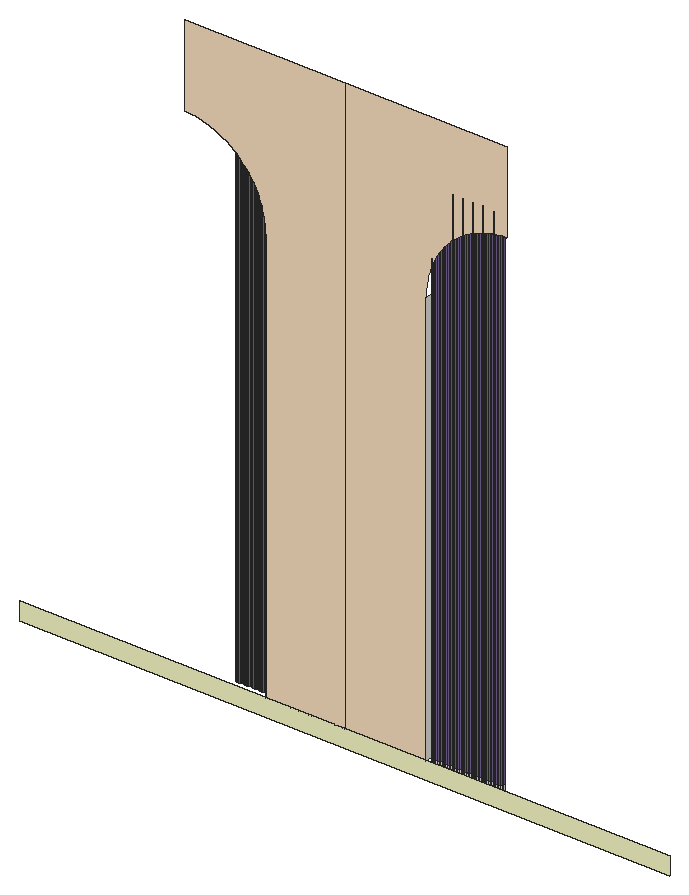
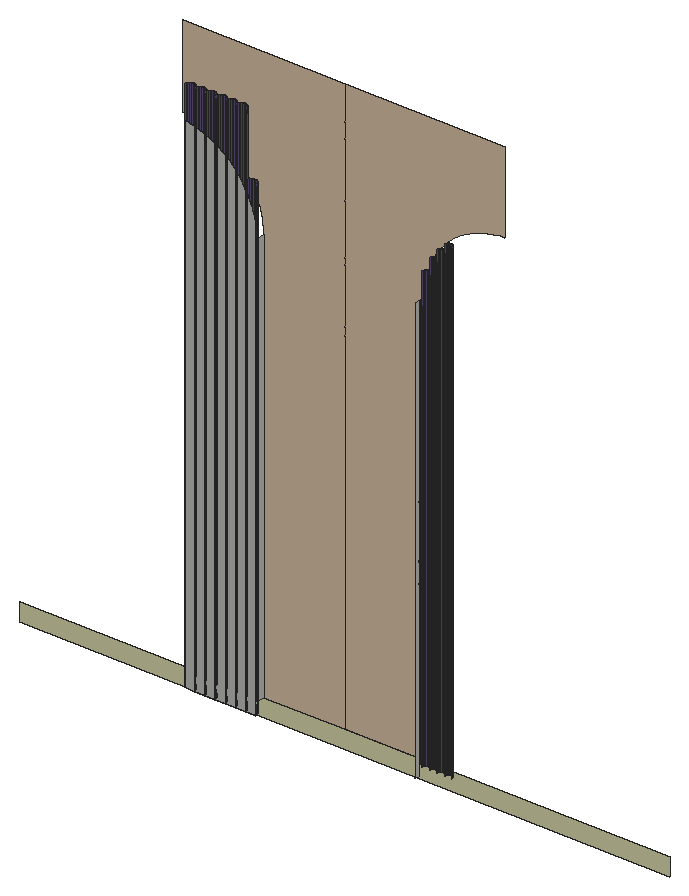
# SketchUp Ruby script. Lengths in inches.
U = 1.inch
M = Sketchup.active_model
def pt(a) = Geom::Point3d.new(a.map { |v| v * U })
def face(e, loops, mat)
  f = e.add_face(loops[0].map { |a| pt(a) })
  loops[1..].each { |l| e.add_face(l.map { |a| pt(a) }).erase! }
  f.material = f.back_material = mat if mat
  f
end
# faces: each face lists its corners as indices into pts; further lists are holes
def faces(e, pts, list, mat = nil) = list.each { |f| face(e, (f[0].is_a?(Array) ? f : [f]).map { |l| l.map { |i| pts[i] } }, mat) }
# xy, xz, yz: faces in a plane at the given z, y or x. An outline is a flat list of corners, or four numbers for a rectangle; further outlines are holes
def ring(l) = l.size == 4 ? [[l[0], l[1]], [l[2], l[1]], [l[2], l[3]], [l[0], l[3]]] : l.each_slice(2).to_a
def flat(e, list, mat, &to3) = list.each { |f| face(e, (f[0].is_a?(Array) ? f : [f]).map { |l| ring(l).map { |u, v| to3.(u, v) } }, mat) }
def xy(e, z, list, mat = nil) = flat(e, list, mat) { |x, y| [x, y, z] }
def xz(e, y, list, mat = nil) = flat(e, list, mat) { |x, z| [x, y, z] }
def yz(e, x, list, mat = nil) = flat(e, list, mat) { |y, z| [x, y, z] }
def lines(e, pts, list) = list.each { |a, b| e.add_line(pt(pts[a]), pt(pts[b])) }
# prism: a flat outline (further loops are holes) pulled along v
def prism(e, loops, v, mat = nil)
  f = face(e, loops, mat); d = Geom::Vector3d.new(v.map { |x| x * U })
  f.pushpull(f.normal.samedirection?(d) ? d.length : -d.length)
end
def box(e, o, s, mat = nil) = prism(e, [[o, [o[0] + s[0], o[1], o[2]], [o[0] + s[0], o[1] + s[1], o[2]], [o[0], o[1] + s[1], o[2]]]], [0, 0, s[2]], mat)
def at(x, y, z, deg = 0) = Geom::Transformation.translation(pt([x, y, z])) * Geom::Transformation.rotation(ORIGIN, Z_AXIS, deg.degrees)
def axes(o, x, y, z) = Geom::Transformation.new([*x, 0, *y, 0, *z, 0, *pt(o).to_a, 1])
def part(name) = M.definitions.add(name)
# library, detail: a bought-in or finely detailed component or shape, given as its bounding box
def library(name, o, s) = part(name).tap { |d| box(d.entities, o, s) }
def detail(e, o, s) = box(e.add_group.entities, o, s)
def put(e, d, t, mat = nil) = e.add_instance(d, t).tap { |i| i.material = mat if mat }
def group(e, t, mat = nil) = e.add_group.tap { |g| g.transformation = t; g.material = mat if mat }.entities
root = M.entities
M.materials.add("[0012_Bisque]").color = [255, 228, 196]
M.materials.add("[Color E01]").color = [255, 255, 204]
M.materials.add("[Color I01]").color = [116, 98, 147]
xy(root,5.5,[[176.942,140.478,176.756,140.503,176.583,140.575,176.434,140.689,176.32,140.838,176.248,141.011,176.224,141.197,177.661,141.197,177.637,141.011,177.565,140.838,177.451,140.689,177.302,140.575,177.128,140.503],[178.38,140.478,178.194,140.503,178.02,140.575,177.872,140.689,177.757,140.838,177.686,141.011,177.661,141.197,179.099,141.197,179.074,141.011,179.002,140.838,178.888,140.689,178.739,140.575,178.566,140.503],[179.817,140.478,179.631,140.503,179.458,140.575,179.309,140.689,179.195,140.838,179.123,141.011,179.099,141.197,180.536,141.197,180.512,141.011,180.44,140.838,180.326,140.689,180.177,140.575,180.003,140.503],[181.255,140.478,181.069,140.503,180.895,140.575,180.747,140.689,180.632,140.838,180.561,141.011,180.536,141.197,181.974,141.197,181.949,141.011,181.877,140.838,181.763,140.689,181.614,140.575,181.441,140.503],[182.692,140.478,182.506,140.503,182.333,140.575,182.184,140.689,182.07,140.838,181.998,141.011,181.974,141.197,183.411,141.197,183.387,141.011,183.315,140.838,183.201,140.689,183.052,140.575,182.878,140.503],
  [184.13,140.478,183.944,140.503,183.77,140.575,183.622,140.689,183.507,140.838,183.436,141.011,183.411,141.197,184.849,141.197,184.824,141.011,184.752,140.838,184.638,140.689,184.489,140.575,184.316,140.503],[185.567,140.478,185.381,140.503,185.208,140.575,185.059,140.689,184.945,140.838,184.873,141.011,184.849,141.197,186.286,141.197,186.262,141.011,186.19,140.838,186.076,140.689,185.927,140.575,185.753,140.503],[153.72,140.735,153.724,140.737,153.834,140.822,153.918,140.932,153.971,141.06,153.989,141.197,153.72,141.197]])
xz(root,139.885,[[153.72,7.1875,164.816,7.1875,164.816,88.4375,142.302,88.4375,142.302,76.971,142.307,76.971,142.612,76.963,142.917,76.947,143.221,76.923,143.525,76.891,143.828,76.851,144.129,76.803,144.429,76.747,144.728,76.683,145.024,76.611,145.319,76.531,145.612,76.444,145.902,76.349,146.189,76.246,146.474,76.136,146.756,76.018,147.034,75.893,147.309,75.761,147.581,75.621,147.848,75.474,148.112,75.321,148.372,75.16,148.627,74.993,148.878,74.818,149.124,74.638,149.365,74.451,149.601,74.257,149.832,74.058,150.058,73.852,150.278,73.64,150.492,73.423,150.701,73.2,150.904,72.972,151.1,72.738,151.291,72.5,151.475,72.256,151.652,72.008,151.823,71.755,151.987,71.497,152.145,71.236,152.295,70.97,152.438,70.7,152.574,70.427,152.703,70.15,152.825,69.87,152.939,69.587,153.045,69.301,153.144,69.012,153.235,68.721,153.319,68.427,153.395,68.132,153.463,67.834,153.523,67.535,153.575,67.234,153.619,66.932,153.655,66.629,153.683,66.325,153.704,66.02,153.716,65.715,153.72,65.41],[164.816,7.1875,176.224,7.1875,176.224,65.41,176.228,65.71,176.239,66.01,176.259,66.309,176.286,66.608,176.321,66.906,176.364,67.203,176.414,67.499,176.472,67.793,176.538,68.086,176.611,68.377,176.692,68.666,176.78,68.953,176.876,69.237,176.979,69.519,177.089,69.798,177.206,70.075,177.331,70.348,177.463,70.617,177.601,70.883,177.747,71.146,177.899,71.405,178.058,71.659,178.224,71.909,178.395,72.155,178.574,72.397,178.758,72.634,178.949,72.865,179.145,73.092,179.347,73.314,179.555,73.53,179.769,73.741,179.988,73.946,180.212,74.146,180.441,74.34,180.676,74.527,180.915,74.709,181.158,74.884,181.406,75.053,181.659,75.215,181.915,75.371,182.176,75.52,182.44,75.662,182.708,75.797,182.979,75.926,183.254,76.047,183.531,76.161,183.812,76.268,184.095,76.367,184.381,76.459,184.669,76.544,184.959,76.621,185.25,76.691,185.544,76.753,185.839,76.807,186.136,76.854,186.433,76.893,186.732,76.924,187.031,76.947,187.331,76.963,187.631,76.952,187.631,88.4375,164.816,88.4375]],"[0012_Bisque]")
xz(root,139.885,[[119.1875,4.6875,210.445,7.1875]],"[Color E01]")
xz(root,141.197,[[176.224,5.5,177.661,5.5,177.661,70.991,177.601,70.883,177.463,70.617,177.331,70.348,177.206,70.075,177.089,69.798,176.979,69.519,176.876,69.237,176.78,68.953,176.692,68.666,176.611,68.377,176.538,68.086,176.472,67.793,176.414,67.499,176.364,67.203,176.321,66.906,176.286,66.608,176.259,66.309,176.239,66.01,176.228,65.71,176.224,65.41],[177.661,5.5,177.661,70.991,177.747,71.146,177.899,71.405,178.058,71.659,178.224,71.909,178.395,72.155,178.574,72.397,178.758,72.634,178.949,72.865,179.099,73.039,179.099,5.5],[179.099,5.5,180.536,5.5,180.536,74.416,180.441,74.34,180.212,74.146,179.988,73.946,179.769,73.741,179.555,73.53,179.347,73.314,179.145,73.092,179.099,73.039],[180.536,5.5,181.974,5.5,181.974,75.404,181.915,75.371,181.659,75.215,181.406,75.053,181.158,74.884,180.915,74.709,180.676,74.527,180.536,74.416],[181.974,5.5,183.411,5.5,183.411,76.111,183.254,76.047,182.979,75.926,182.708,75.797,182.44,75.662,182.176,75.52,181.974,75.404],
  [183.411,5.5,184.849,5.5,184.849,76.592,184.669,76.544,184.381,76.459,184.095,76.367,183.812,76.268,183.531,76.161,183.411,76.111],[184.849,5.5,186.286,5.5,186.286,76.873,186.136,76.854,185.839,76.807,185.544,76.753,185.25,76.691,184.959,76.621,184.849,76.592]])
yz(root,153.72,[[140.735,5.5,141.197,65.41],[139.885,7.1875,140.735,65.41]])
yz(root,176.224,[[139.885,7.1875,141.197,65.41]])
p = [[176.583,140.575,5.5],[176.756,140.503,5.5],[176.756,140.503,7.1875],[176.583,140.575,7.1875],[176.942,140.478,5.5],[176.942,140.478,7.1875],
  [177.128,140.503,5.5],[177.128,140.503,7.1875],[177.302,140.575,5.5],[177.302,140.575,7.1875],[178.02,140.575,5.5],[178.194,140.503,5.5],
  [178.194,140.503,7.1875],[178.02,140.575,7.1875],[178.38,140.478,5.5],[178.38,140.478,7.1875],[178.566,140.503,5.5],[178.566,140.503,7.1875],
  [178.739,140.575,5.5],[178.739,140.575,7.1875],[179.458,140.575,5.5],[179.631,140.503,5.5],[179.631,140.503,7.1875],[179.458,140.575,7.1875],
  [179.817,140.478,5.5],[179.817,140.478,7.1875],[180.003,140.503,5.5],[180.003,140.503,7.1875],[180.177,140.575,5.5],[180.177,140.575,7.1875],
  [180.895,140.575,5.5],[181.069,140.503,5.5],[181.069,140.503,7.1875],[180.895,140.575,7.1875],[181.255,140.478,5.5],[181.255,140.478,7.1875],
  [181.441,140.503,5.5],[181.441,140.503,7.1875],[181.614,140.575,5.5],[181.614,140.575,7.1875],[182.333,140.575,5.5],[182.506,140.503,5.5],
  [182.506,140.503,7.1875],[182.333,140.575,7.1875],[182.692,140.478,5.5],[182.692,140.478,7.1875],[182.878,140.503,5.5],[182.878,140.503,7.1875],
  [183.052,140.575,5.5],[183.052,140.575,7.1875],[183.77,140.575,5.5],[183.944,140.503,5.5],[183.944,140.503,7.1875],[183.77,140.575,7.1875],
  [184.13,140.478,5.5],[184.13,140.478,7.1875],[184.316,140.503,5.5],[184.316,140.503,7.1875],[184.489,140.575,5.5],[184.489,140.575,7.1875],
  [185.208,140.575,5.5],[185.381,140.503,5.5],[185.381,140.503,7.1875],[185.208,140.575,7.1875],[185.567,140.478,5.5],[185.567,140.478,7.1875],
  [185.753,140.503,5.5],[185.753,140.503,7.1875],[185.927,140.575,5.5],[185.927,140.575,7.1875],[176.434,140.689,5.5],[176.434,140.689,7.1875],
  [177.451,140.689,5.5],[177.451,140.689,7.1875],[177.872,140.689,5.5],[177.872,140.689,7.1875],[178.888,140.689,5.5],[178.888,140.689,7.1875],
  [179.309,140.689,5.5],[179.309,140.689,7.1875],[180.326,140.689,5.5],[180.326,140.689,7.1875],[180.747,140.689,5.5],[180.747,140.689,7.1875],
  [181.763,140.689,5.5],[181.763,140.689,7.1875],[182.184,140.689,5.5],[182.184,140.689,7.1875],[183.201,140.689,5.5],[183.201,140.689,7.1875],
  [183.622,140.689,5.5],[183.622,140.689,7.1875],[184.638,140.689,5.5],[184.638,140.689,7.1875],[185.059,140.689,5.5],[185.059,140.689,7.1875],
  [186.076,140.689,5.5],[186.076,140.689,7.1875],[176.32,140.838,5.5],[176.32,140.838,7.1875],[177.565,140.838,5.5],[177.565,140.838,7.1875],
  [177.757,140.838,5.5],[177.757,140.838,7.1875],[179.002,140.838,5.5],[179.002,140.838,7.1875],[179.195,140.838,5.5],[179.195,140.838,7.1875],
  [180.44,140.838,5.5],[180.44,140.838,7.1875],[180.632,140.838,5.5],[180.632,140.838,7.1875],[181.877,140.838,5.5],[181.877,140.838,7.1875],
  [182.07,140.838,5.5],[182.07,140.838,7.1875],[183.315,140.838,5.5],[183.315,140.838,7.1875],[183.507,140.838,5.5],[183.507,140.838,7.1875],
  [184.752,140.838,5.5],[184.752,140.838,7.1875],[184.945,140.838,5.5],[184.945,140.838,7.1875],[186.19,140.838,5.5],[186.19,140.838,7.1875],
  [176.248,141.011,7.1875],[176.248,141.011,5.5],[177.637,141.011,5.5],[177.637,141.011,7.1875],[177.686,141.011,5.5],[177.686,141.011,7.1875],
  [179.074,141.011,5.5],[179.074,141.011,7.1875],[179.123,141.011,5.5],[179.123,141.011,7.1875],[180.512,141.011,5.5],[180.512,141.011,7.1875],
  [180.561,141.011,5.5],[180.561,141.011,7.1875],[181.949,141.011,5.5],[181.949,141.011,7.1875],[181.998,141.011,5.5],[181.998,141.011,7.1875],
  [183.387,141.011,5.5],[183.387,141.011,7.1875],[183.436,141.011,5.5],[183.436,141.011,7.1875],[184.824,141.011,5.5],[184.824,141.011,7.1875],
  [184.873,141.011,5.5],[184.873,141.011,7.1875],[186.262,141.011,5.5],[186.262,141.011,7.1875],[176.224,141.197,5.5],[176.224,141.197,7.1875],
  [177.661,141.197,5.5],[177.661,141.197,7.1875],[179.099,141.197,5.5],[179.099,141.197,7.1875],[180.536,141.197,5.5],[180.536,141.197,7.1875],
  [181.974,141.197,5.5],[181.974,141.197,7.1875],[183.411,141.197,5.5],[183.411,141.197,7.1875],[184.849,141.197,5.5],[184.849,141.197,7.1875],
  [186.286,141.197,5.5],[186.286,141.197,7.1875],[176.583,140.575,72.397],[176.756,140.503,72.397],[176.942,140.478,72.397],[177.128,140.503,72.397],
  [177.302,140.575,72.397],[178.02,140.575,81.5],[178.194,140.503,81.5],[178.38,140.478,81.5],[178.566,140.503,81.5],[178.739,140.575,81.5],
  [179.458,140.575,81.5],[179.631,140.503,81.5],[179.817,140.478,81.5],[180.003,140.503,81.5],[180.177,140.575,81.5],[180.895,140.575,81.5],
  [181.069,140.503,81.5],[181.255,140.478,81.5],[181.441,140.503,81.5],[181.614,140.575,81.5],[182.333,140.575,81.5],[182.506,140.503,81.5],
  [182.692,140.478,81.5],[182.878,140.503,81.5],[183.052,140.575,81.5],[183.77,140.575,81.5],[183.944,140.503,81.5],[184.13,140.478,81.5],
  [184.316,140.503,81.5],[184.489,140.575,81.5],[185.208,140.575,81.5],[185.381,140.503,81.5],[185.567,140.478,81.5],[185.753,140.503,81.5],
  [185.927,140.575,81.5],[176.434,140.689,72.397],[177.451,140.689,72.397],[177.872,140.689,81.5],[178.888,140.689,81.5],[179.309,140.689,81.5],
  [180.326,140.689,81.5],[180.747,140.689,81.5],[181.763,140.689,81.5],[182.184,140.689,81.5],[183.201,140.689,81.5],[183.622,140.689,81.5],
  [184.638,140.689,81.5],[185.059,140.689,81.5],[186.076,140.689,81.5],[148.833,140.822,74.138],[148.833,140.822,7.1875],[148.943,140.737,7.1875],
  [148.943,140.737,74.138],[149.071,140.684,7.1875],[149.071,140.684,74.138],[149.208,140.666,7.1875],[149.208,140.666,74.138],[149.346,140.684,7.1875],
  [149.346,140.684,74.138],[149.474,140.737,7.1875],[149.474,140.737,74.138],[149.584,140.822,7.1875],[149.584,140.822,74.138],[149.895,140.822,73.087],
  [149.895,140.822,7.1875],[150.005,140.737,7.1875],[150.005,140.737,73.087],[150.133,140.684,7.1875],[150.133,140.684,73.087],[150.271,140.666,7.1875],
  [150.271,140.666,73.087],[150.408,140.684,7.1875],[150.408,140.684,73.087],[150.536,140.737,7.1875],[150.536,140.737,73.087],[150.646,140.822,7.1875],
  [150.646,140.822,73.087],[150.958,140.822,71.69],[150.958,140.822,7.1875],[151.068,140.737,7.1875],[151.068,140.737,71.69],[151.196,140.684,7.1875],
  [151.196,140.684,71.69],[151.333,140.666,7.1875],[151.333,140.666,71.69],[151.471,140.684,7.1875],[151.471,140.684,71.69],[151.599,140.737,7.1875],
  [151.599,140.737,71.69],[151.709,140.822,7.1875],[151.709,140.822,71.69],[152.02,140.822,69.616],[152.02,140.822,7.1875],[152.13,140.737,7.1875],
  [152.13,140.737,69.616],[152.258,140.684,7.1875],[152.258,140.684,69.616],[152.396,140.666,7.1875],[152.396,140.666,69.616],[152.533,140.684,7.1875],
  [152.533,140.684,69.616],[152.661,140.737,7.1875],[152.661,140.737,69.616],[152.771,140.822,7.1875],[152.771,140.822,69.616],[153.083,140.822,65.41],
  [153.083,140.822,7.1875],[153.193,140.737,7.1875],[153.193,140.737,65.41],[153.321,140.684,7.1875],[153.321,140.684,65.41],[153.458,140.666,7.1875],
  [153.458,140.666,65.41],[153.596,140.684,7.1875],[153.596,140.684,65.41],[153.72,140.735,7.1875],[153.72,140.735,65.41],[176.32,140.838,66.906],
  [176.32,140.838,72.397],[177.565,140.838,72.397],[177.757,140.838,81.5],[179.002,140.838,81.5],[179.195,140.838,81.5],[180.44,140.838,81.5],
  [180.632,140.838,81.5],[181.877,140.838,81.5],[182.07,140.838,81.5],[183.315,140.838,81.5],[183.507,140.838,81.5],[184.752,140.838,81.5],
  [184.945,140.838,81.5],[186.19,140.838,81.5],[148.748,140.932,74.138],[148.748,140.932,7.1875],[149.668,140.932,7.1875],[149.668,140.932,74.138],
  [149.811,140.932,73.087],[149.811,140.932,7.1875],[150.731,140.932,7.1875],[150.731,140.932,73.087],[150.873,140.932,71.69],[150.873,140.932,7.1875],
  [151.793,140.932,7.1875],[151.793,140.932,71.69],[151.936,140.932,69.616],[151.936,140.932,7.1875],[152.856,140.932,7.1875],[152.856,140.932,69.616],
  [152.998,140.932,65.41],[152.998,140.932,7.1875],[176.248,141.011,72.397],[177.637,141.011,72.397],[177.686,141.011,81.5],[179.074,141.011,81.5],
  [179.123,141.011,81.5],[180.512,141.011,81.5],[180.561,141.011,81.5],[181.949,141.011,81.5],[181.998,141.011,81.5],[183.387,141.011,81.5],
  [183.436,141.011,81.5],[184.824,141.011,81.5],[184.873,141.011,81.5],[186.262,141.011,81.5],[148.695,141.06,74.138],[148.695,141.06,7.1875],
  [149.721,141.06,7.1875],[149.721,141.06,74.138],[149.758,141.06,73.087],[149.758,141.06,7.1875],[150.784,141.06,7.1875],[150.784,141.06,73.087],
  [150.82,141.06,71.69],[150.82,141.06,7.1875],[151.846,141.06,7.1875],[151.846,141.06,71.69],[151.883,141.06,69.616],[151.883,141.06,7.1875],
  [152.909,141.06,7.1875],[152.909,141.06,69.616],[152.945,141.06,65.41],[152.945,141.06,7.1875],[176.224,141.197,65.41],[176.224,141.197,72.397],
  [177.661,141.197,70.991],[177.661,141.197,72.397],[177.661,141.197,81.5],[179.099,141.197,73.039],[179.099,141.197,81.5],[180.536,141.197,74.416],
  [180.536,141.197,81.5],[181.974,141.197,75.404],[181.974,141.197,81.5],[183.411,141.197,76.111],[183.411,141.197,81.5],[184.849,141.197,76.592],
  [184.849,141.197,81.5],[186.286,141.197,76.873],[186.286,141.197,81.5],[148.677,141.197,74.138],[148.677,141.197,7.1875],[149.739,141.197,7.1875],
  [149.739,141.197,73.087],[149.739,141.197,74.138],[150.802,141.197,7.1875],[150.802,141.197,71.69],[150.802,141.197,73.003],[150.802,141.197,73.087],
  [151.864,141.197,7.1875],[151.864,141.197,69.616],[151.864,141.197,71.69],[152.927,141.197,7.1875],[152.927,141.197,65.41],[152.927,141.197,66.722],
  [152.927,141.197,69.616]]
faces(root,p,[[0,1,2,3],[1,4,5,2],[4,6,7,5],[6,8,9,7],[10,11,12,13],[11,14,15,12],[14,16,17,15],[16,18,19,17],
  [20,21,22,23],[21,24,25,22],[24,26,27,25],[26,28,29,27],[30,31,32,33],[31,34,35,32],[34,36,37,35],[36,38,39,37],
  [40,41,42,43],[41,44,45,42],[44,46,47,45],[46,48,49,47],[50,51,52,53],[51,54,55,52],[54,56,57,55],[56,58,59,57],
  [60,61,62,63],[61,64,65,62],[64,66,67,65],[66,68,69,67],[70,0,3,71],[8,72,73,9],[74,10,13,75],[18,76,77,19],
  [78,20,23,79],[28,80,81,29],[82,30,33,83],[38,84,85,39],[86,40,43,87],[48,88,89,49],[90,50,53,91],[58,92,93,59],
  [94,60,63,95],[68,96,97,69],[98,70,71,99],[72,100,101,73],[102,74,75,103],[76,104,105,77],[106,78,79,107],[80,108,109,81],
  [110,82,83,111],[84,112,113,85],[114,86,87,115],[88,116,117,89],[118,90,91,119],[92,120,121,93],[122,94,95,123],[96,124,125,97],
  [98,99,126,127],[100,128,129,101],[130,102,103,131],[104,132,133,105],[134,106,107,135],[108,136,137,109],[138,110,111,139],[112,140,141,113],
  [142,114,115,143],[116,144,145,117],[146,118,119,147],[120,148,149,121],[150,122,123,151],[124,152,153,125],[154,127,126,155],[128,156,157,129],
  [156,130,131,157],[132,158,159,133],[158,134,135,159],[136,160,161,137],[160,138,139,161],[140,162,163,141],[162,142,143,163],[144,164,165,145],
  [164,146,147,165],[148,166,167,149],[166,150,151,167],[152,168,169,153]])
faces(root,p,[[170,3,2,171],[171,2,5,172],[172,5,7,173],[173,7,9,174],[175,13,12,176],[176,12,15,177],[177,15,17,178],[178,17,19,179],
  [180,23,22,181],[181,22,25,182],[182,25,27,183],[183,27,29,184],[185,33,32,186],[186,32,35,187],[187,35,37,188],[188,37,39,189],
  [190,43,42,191],[191,42,45,192],[192,45,47,193],[193,47,49,194],[195,53,52,196],[196,52,55,197],[197,55,57,198],[198,57,59,199],
  [200,63,62,201],[201,62,65,202],[202,65,67,203],[203,67,69,204],[205,71,3,170],[174,9,73,206],[207,75,13,175],[179,19,77,208],
  [209,79,23,180],[184,29,81,210],[211,83,33,185],[189,39,85,212],[213,87,43,190],[194,49,89,214],[215,91,53,195],[199,59,93,216],
  [217,95,63,200],[204,69,97,218],[219,220,221,222],[222,221,223,224],[224,223,225,226],[226,225,227,228],[228,227,229,230],[230,229,231,232],
  [233,234,235,236],[236,235,237,238],[238,237,239,240],[240,239,241,242],[242,241,243,244],[244,243,245,246],[247,248,249,250],[250,249,251,252],
  [252,251,253,254],[254,253,255,256],[256,255,257,258],[258,257,259,260],[261,262,263,264],[264,263,265,266],[266,265,267,268],[268,267,269,270],
  [270,269,271,272],[272,271,273,274],[275,276,277,278],[278,277,279,280],[280,279,281,282],[282,281,283,284],[284,283,285,286],[287,99,71,205,288],
  [206,73,101,289],[290,103,75,207],[208,77,105,291],[292,107,79,209],[210,81,109,293],[294,111,83,211],[212,85,113,295],[296,115,87,213],
  [214,89,117,297],[298,119,91,215],[216,93,121,299],[300,123,95,217],[218,97,125,301],[302,303,220,219],[232,231,304,305],[306,307,234,233],
  [246,245,308,309],[310,311,248,247],[260,259,312,313],[314,315,262,261],[274,273,316,317],[318,319,276,275],[320,126,99,287,288],[289,101,129,321],
  [322,131,103,290],[291,105,133,323],[324,135,107,292],[293,109,137,325],[326,139,111,294],[295,113,141,327],[328,143,115,296],[297,117,145,329],
  [330,147,119,298],[299,121,149,331],[332,151,123,300],[301,125,153,333],[334,335,303,302],[305,304,336,337],[338,339,307,306],[309,308,340,341],
  [342,343,311,310],[313,312,344,345],[346,347,315,314],[317,316,348,349],[350,351,319,318],[352,155,126,320,353],[321,129,157,354,355],[354,157,131,322,356,355],
  [323,133,159,357,358],[357,159,135,324,358],[325,137,161,359,360],[359,161,139,326,360],[327,141,163,361,362],[361,163,143,328,362],[329,145,165,363,364],[363,165,147,330,364],
  [331,149,167,365,366],[365,167,151,332,366],[333,153,169,367,368],[369,370,335,334],[337,336,371,372,373],[372,371,339,338],[341,340,374,375,376,377],[375,374,343,342],
  [345,344,378,379,380],[379,378,347,346],[349,348,381,382,383,384],[382,381,351,350]],"[Color I01]")
